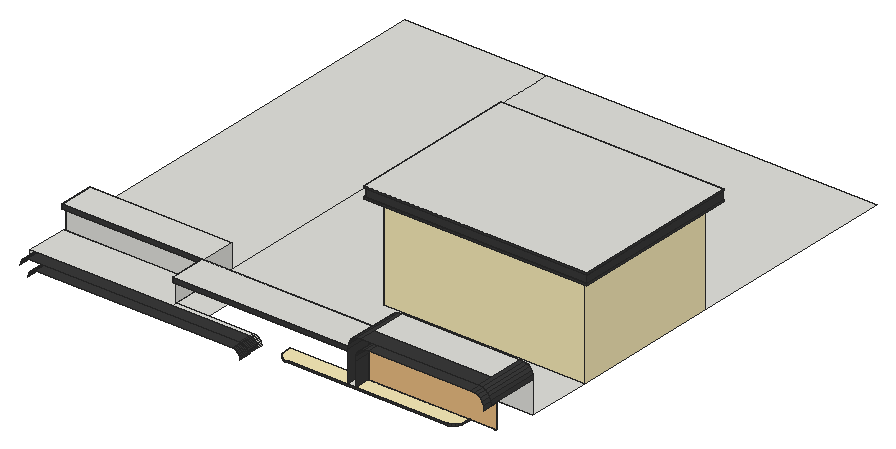
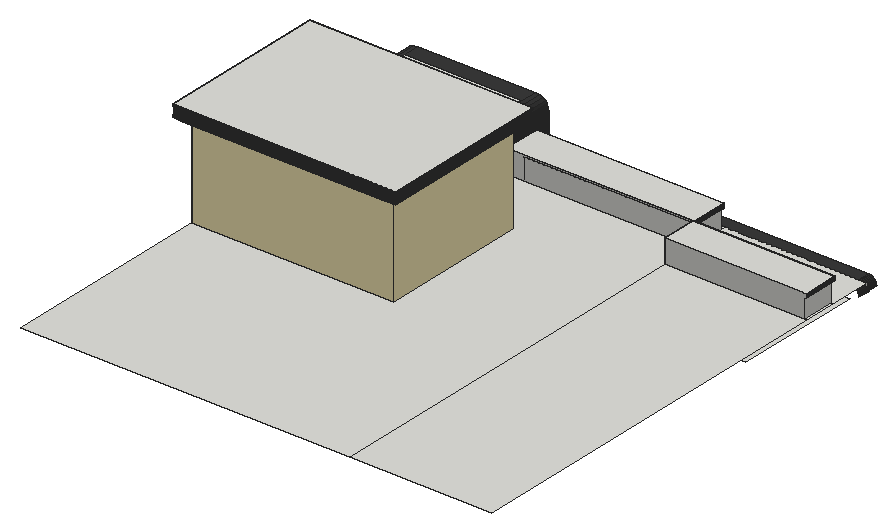
# SketchUp Ruby script. Lengths in inches.
U = 1.inch
M = Sketchup.active_model
def pt(a) = Geom::Point3d.new(a.map { |v| v * U })
def face(e, loops, mat)
  f = e.add_face(loops[0].map { |a| pt(a) })
  loops[1..].each { |l| e.add_face(l.map { |a| pt(a) }).erase! }
  f.material = f.back_material = mat if mat
  f
end
# faces: each face lists its corners as indices into pts; further lists are holes
def faces(e, pts, list, mat = nil) = list.each { |f| face(e, (f[0].is_a?(Array) ? f : [f]).map { |l| l.map { |i| pts[i] } }, mat) }
# xy, xz, yz: faces in a plane at the given z, y or x. An outline is a flat list of corners, or four numbers for a rectangle; further outlines are holes
def ring(l) = l.size == 4 ? [[l[0], l[1]], [l[2], l[1]], [l[2], l[3]], [l[0], l[3]]] : l.each_slice(2).to_a
def flat(e, list, mat, &to3) = list.each { |f| face(e, (f[0].is_a?(Array) ? f : [f]).map { |l| ring(l).map { |u, v| to3.(u, v) } }, mat) }
def xy(e, z, list, mat = nil) = flat(e, list, mat) { |x, y| [x, y, z] }
def xz(e, y, list, mat = nil) = flat(e, list, mat) { |x, z| [x, y, z] }
def yz(e, x, list, mat = nil) = flat(e, list, mat) { |y, z| [x, y, z] }
def lines(e, pts, list) = list.each { |a, b| e.add_line(pt(pts[a]), pt(pts[b])) }
# prism: a flat outline (further loops are holes) pulled along v
def prism(e, loops, v, mat = nil)
  f = face(e, loops, mat); d = Geom::Vector3d.new(v.map { |x| x * U })
  f.pushpull(f.normal.samedirection?(d) ? d.length : -d.length)
end
def box(e, o, s, mat = nil) = prism(e, [[o, [o[0] + s[0], o[1], o[2]], [o[0] + s[0], o[1] + s[1], o[2]], [o[0], o[1] + s[1], o[2]]]], [0, 0, s[2]], mat)
def at(x, y, z, deg = 0) = Geom::Transformation.translation(pt([x, y, z])) * Geom::Transformation.rotation(ORIGIN, Z_AXIS, deg.degrees)
def axes(o, x, y, z) = Geom::Transformation.new([*x, 0, *y, 0, *z, 0, *pt(o).to_a, 1])
def part(name) = M.definitions.add(name)
# library, detail: a bought-in or finely detailed component or shape, given as its bounding box
def library(name, o, s) = part(name).tap { |d| box(d.entities, o, s) }
def detail(e, o, s) = box(e.add_group.entities, o, s)
def put(e, d, t, mat = nil) = e.add_instance(d, t).tap { |i| i.material = mat if mat }
def group(e, t, mat = nil) = e.add_group.tap { |g| g.transformation = t; g.material = mat if mat }.entities
root = M.entities
M.materials.add("0899 AP 7833 SUNKISSED").color = [249, 236, 185]
M.materials.add("[Color M07]").color = [58, 58, 58]
M.materials.add("[Wood Veneer 02]").color = [190, 128, 91]
c1 = library("Group277\#1",[-65.14,-19,0],[130.28,38,0.24])
xy(root,243,[[9,135.1875,166.1,267.1875]])
xy(root,247,[[17,111.1875,217,123.1875]],"[Color M07]")
xy(root,253.0625,[[274.28,111.1875,432.47,111.1875,436.3,111.52,439.43,112.52,441.87,114.1875,443.61,116.52,444.65,119.52,445,123.1875,261.75,123.1875,262.1,119.52,263.14,116.52,264.88,114.1875,267.32,112.52,270.45,111.52]])
xy(root,255,[[334.71,111.1875,342.71,128.1875],[1,123.1875,145.5625,166.1875],[145.5625,123.1875,225,128.1875],[145.5625,164.1875,481,164.1875,481,230.0625,275.625,230.0625,275.625,382.59,481,382.59,481,601,145.5625,601],[1,166.1875,3,200.1875],
  [3,166.1875,145.5625,200.1875],[1,200.1875,145.5625,601],[275.625,230.0625,481,382.59]])
xy(root,255,[[274.28,111.1875,334.71,111.1875,334.71,128.1875,261.75,128.1875,261.75,123.1875,262.1,119.52,263.14,116.52,264.88,114.1875,267.32,112.52,270.45,111.52],[342.71,111.1875,432.47,111.1875,436.3,111.52,439.43,112.52,441.87,114.1875,443.61,116.52,444.65,119.52,445,123.1875,445,128.1875,342.71,128.1875]],"0899 AP 7833 SUNKISSED")
xy(root,255,[[9,111.1875,225,123.1875]],"[Color M07]")
xy(root,274.625,[[145.39,126.1875,144.83,126.24,144.37,126.39,144.02,126.64,143.77,127,143.61,127.45,143.5625,128.01,143.5625,164.1875,145.5625,164.1875,145.5625,128.1875,334.71,128.1875,334.71,126.1875],[1,164.1875,143.5625,166.1875],[143.5625,164.1875,145.5625,166.1875],[1,166.1875,3,200.1875]],"[Color M07]")
xy(root,277,[[145.5625,128.1875,317.59,164.1875]])
xy(root,279,[[145.39,126.1875,334.71,126.1875,334.71,164.1875,143.5625,164.1875,143.5625,128.01,143.61,127.45,143.77,127,144.02,126.64,144.37,126.39,144.83,126.24],[1,164.1875,145.5625,200.1875]])
xy(root,293,[[356.2,111.1875,459.51,128.1875]],"[Color M07]")
xy(root,301,[[348.2,128.1875,467.51,164.1875]])
xy(root,301,[[348.2,111.1875,467.51,128.1875]],"[Color M07]")
xy(root,352.4375,[[275.625,230.0625,481,382.59],[275.625,382.59,481,393.59]])
xy(root,352.4375,[[264.625,219.0625,264.625,393.59,275.625,393.59,275.625,230.0625,481,230.0625,481,393.59,492,393.59,492,219.0625]],"[Color M07]")
xy(root,354.4375,[[265.625,220.0625,491,392.59]])
xy(root,354.4375,[[264.625,219.0625,492,220.0625],[264.625,220.0625,265.625,393.59],[491,220.0625,492,393.59],[265.625,392.59,491,393.59]],"[Color M07]")
xy(root,362.4375,[[265.625,220.0625,491,392.59]])
xy(root,362.4375,[[264.625,219.0625,492,220.0625],[264.625,220.0625,265.625,393.59],[491,220.0625,492,393.59],[265.625,392.59,491,393.59]],"[Color M07]")
xy(root,364.4375,[[264.625,219.0625,492,393.59]])
xz(root,111.1875,[[274.28,253.0625,432.47,255]],"[Color M07]")
xz(root,123.1875,[[1,247,1.07,248.04,1.27,249.07,1.61,250.0625,2.07,251,2.65,251.87,3.34,252.66,4.13,253.35,5,253.93,5.9375,254.39,6.93,254.73,7.96,254.93,9,255,1,255]])
xz(root,126.1875,[[145.39,274.625,334.71,279]],"[Color M07]")
xz(root,128.1875,[[145.5625,274.625,317.59,277]])
xz(root,164.1875,[[145.5625,255,317.59,277],[317.59,255,317.59,279,334.71,279,334.71,287.51,335.09,291.63,336.21,295.01,338.08,297.63,340.71,299.5,344.08,300.625,348.2,301,467.51,301,471.63,300.625,475.01,299.5,477.63,297.63,479.5,295.01,480.625,291.63,481,287.51,481,255],[143.5625,274.625,145.5625,279],[145.5625,277,317.59,279]])
xz(root,164.1875,[[1,274.625,143.5625,279]],"[Color M07]")
xz(root,166.1875,[[3,255,145.5625,274.625]])
xz(root,200.1875,[[3,255,3,274.625,1,274.625,1,279,145.5625,279,145.5625,255]])
xz(root,219.0625,[[264.625,352.4375,492,354.4375],[264.625,362.4375,492,364.4375]],"[Color M07]")
xz(root,220.0625,[[265.625,354.4375,491,362.4375]],"[Color M07]")
xz(root,230.0625,[[275.625,255,481,352.4375]],"0899 AP 7833 SUNKISSED")
xz(root,382.59,[[275.625,255,481,352.4375]],"0899 AP 7833 SUNKISSED")
xz(root,392.59,[[265.625,354.4375,491,362.4375]],"[Color M07]")
xz(root,393.59,[[264.625,352.4375,492,354.4375],[264.625,362.4375,492,364.4375]],"[Color M07]")
yz(root,1,[[164.1875,274.625,200.1875,279]],"[Color M07]")
yz(root,3,[[166.1875,255,200.1875,274.625]])
yz(root,143.5625,[[128.01,274.625,164.1875,279]],"[Color M07]")
yz(root,145.5625,[[128.1875,255,164.1875,274.625],[164.1875,255,166.1875,274.625],[166.1875,255,200.1875,255,200.1875,279,164.1875,279,164.1875,274.625,166.1875,274.625],[128.1875,274.625,164.1875,277]])
yz(root,261.75,[[123.1875,253.0625,128.1875,255]],"[Color M07]")
yz(root,264.625,[[219.0625,352.4375,393.59,354.4375],[219.0625,362.4375,393.59,364.4375]],"[Color M07]")
yz(root,265.625,[[220.0625,354.4375,392.59,362.4375]],"[Color M07]")
yz(root,275.625,[[230.0625,255,382.59,352.4375]],"0899 AP 7833 SUNKISSED")
yz(root,334.71,[[126.1875,274.625,128.1875,279]])
yz(root,334.71,[[111.1875,255,111.1875,287.51,164.1875,287.51,164.1875,279,126.1875,279,126.1875,274.625,128.1875,274.625,128.1875,255]],"[Color M07]")
yz(root,342.71,[[111.1875,255,128.1875,279.51]],"[Color M07]")
yz(root,445,[[123.1875,253.0625,128.1875,255]],"[Color M07]")
yz(root,481,[[230.0625,255,382.59,352.4375]],"0899 AP 7833 SUNKISSED")
yz(root,491,[[220.0625,354.4375,392.59,362.4375]],"[Color M07]")
yz(root,492,[[219.0625,352.4375,393.59,354.4375],[219.0625,362.4375,393.59,364.4375]],"[Color M07]")
p = [[9,123.1875,239],[9.07,123.1875,240.04],[9.07,111.1875,240.04],[9,111.1875,239],[224.93,123.1875,240.04],[225,123.1875,239],
  [225,111.1875,239],[224.93,111.1875,240.04],[9.27,123.1875,241.07],[9.27,111.1875,241.07],[224.73,123.1875,241.07],[224.73,111.1875,241.07],
  [9.61,123.1875,242.0625],[9.61,111.1875,242.0625],[224.39,123.1875,242.0625],[224.39,111.1875,242.0625],[10.07,123.1875,243],[10.07,111.1875,243],
  [223.93,123.1875,243],[223.93,111.1875,243],[10.65,123.1875,243.87],[10.65,111.1875,243.87],[223.35,123.1875,243.87],[223.35,111.1875,243.87],
  [11.34,123.1875,244.66],[11.34,111.1875,244.66],[222.66,123.1875,244.66],[222.66,111.1875,244.66],[12.13,123.1875,245.35],[12.13,111.1875,245.35],
  [221.87,123.1875,245.35],[221.87,111.1875,245.35],[13,123.1875,245.93],[13,111.1875,245.93],[221,123.1875,245.93],[221,111.1875,245.93],
  [13.9375,123.1875,246.39],[13.9375,111.1875,246.39],[220.0625,123.1875,246.39],[220.0625,111.1875,246.39],[14.93,123.1875,246.73],[14.93,111.1875,246.73],
  [219.07,123.1875,246.73],[219.07,111.1875,246.73],[15.96,123.1875,246.93],[15.96,111.1875,246.93],[218.04,123.1875,246.93],[218.04,111.1875,246.93],
  [17,123.1875,247],[17,111.1875,247],[217,123.1875,247],[217,111.1875,247],[1.07,123.1875,248.04],[1,123.1875,247],
  [1,111.1875,247],[1.07,111.1875,248.04],[233,123.1875,247],[232.93,123.1875,248.04],[232.93,111.1875,248.04],[233,111.1875,247],
  [233,128.1875,247],[232.93,128.1875,248.04],[1.27,123.1875,249.07],[1.27,111.1875,249.07],[232.73,123.1875,249.07],[232.73,111.1875,249.07],
  [232.73,128.1875,249.07],[1.61,123.1875,250.0625],[1.61,111.1875,250.0625],[232.39,123.1875,250.0625],[232.39,111.1875,250.0625],[232.39,128.1875,250.0625],
  [2.07,123.1875,251],[2.07,111.1875,251],[231.93,123.1875,251],[231.93,111.1875,251],[231.93,128.1875,251],[2.65,123.1875,251.87],
  [2.65,111.1875,251.87],[231.35,123.1875,251.87],[231.35,111.1875,251.87],[231.35,128.1875,251.87],[3.34,123.1875,252.66],[3.34,111.1875,252.66],
  [230.66,123.1875,252.66],[230.66,111.1875,252.66],[230.66,128.1875,252.66],[4.13,123.1875,253.35],[4.13,111.1875,253.35],[229.87,123.1875,253.35],
  [229.87,111.1875,253.35],[229.87,128.1875,253.35],[270.45,111.52,255],[270.45,111.52,253.0625],[274.28,111.1875,253.0625],[274.28,111.1875,255],
  [432.47,111.1875,255],[432.47,111.1875,253.0625],[436.3,111.52,253.0625],[436.3,111.52,255],[267.32,112.52,255],[267.32,112.52,253.0625],
  [439.43,112.52,253.0625],[439.43,112.52,255],[264.88,114.1875,255],[264.88,114.1875,253.0625],[441.87,114.1875,253.0625],[441.87,114.1875,255],
  [263.14,116.52,255],[263.14,116.52,253.0625],[443.61,116.52,253.0625],[443.61,116.52,255],[262.1,119.52,255],[262.1,119.52,253.0625],
  [444.65,119.52,253.0625],[444.65,119.52,255],[261.75,123.1875,255],[261.75,123.1875,253.0625],[445,123.1875,253.0625],[445,123.1875,255],
  [5,123.1875,253.93],[5,111.1875,253.93],[229,123.1875,253.93],[229,111.1875,253.93],[229,128.1875,253.93],[5.9375,123.1875,254.39],
  [5.9375,111.1875,254.39],[228.0625,123.1875,254.39],[228.0625,111.1875,254.39],[228.0625,128.1875,254.39],[6.93,123.1875,254.73],[6.93,111.1875,254.73],
  [227.07,123.1875,254.73],[227.07,111.1875,254.73],[227.07,128.1875,254.73],[7.96,123.1875,254.93],[7.96,111.1875,254.93],[226.04,123.1875,254.93],
  [226.04,111.1875,254.93],[226.04,128.1875,254.93],[9,123.1875,255],[9,111.1875,255],[225,123.1875,255],[225,111.1875,255],
  [225,128.1875,255],[144.37,126.39,279],[144.37,126.39,274.625],[144.83,126.24,274.625],[144.83,126.24,279],[145.39,126.1875,274.625],
  [145.39,126.1875,279],[144.02,126.64,279],[144.02,126.64,274.625],[143.77,127,279],[143.77,127,274.625],[143.61,127.45,279],
  [143.61,127.45,274.625],[143.5625,128.01,279],[143.5625,128.01,274.625],[342.71,111.1875,279.51],[342.71,128.1875,279.51],[343.09,128.1875,283.63],
  [343.09,111.1875,283.63],[472.625,111.1875,283.63],[472.625,128.1875,283.63],[473,128.1875,279.51],[473,111.1875,279.51],[344.21,128.1875,287.01],
  [344.21,111.1875,287.01],[471.5,111.1875,287.01],[471.5,128.1875,287.01],[346.08,128.1875,289.63],[346.08,111.1875,289.63],[469.63,111.1875,289.63],
  [469.63,128.1875,289.63],[334.71,164.1875,287.51],[334.71,111.1875,287.51],[335.09,111.1875,291.63],[335.09,164.1875,291.63],[480.625,164.1875,291.63],
  [480.625,111.1875,291.63],[481,111.1875,287.51],[481,128.1875,287.51],[481,164.1875,287.51],[348.71,128.1875,291.5],[348.71,111.1875,291.5],
  [467.01,111.1875,291.5],[467.01,128.1875,291.5],[352.08,128.1875,292.625],[352.08,111.1875,292.625],[463.63,111.1875,292.625],[463.63,128.1875,292.625],
  [336.21,111.1875,295.01],[336.21,164.1875,295.01],[479.5,164.1875,295.01],[479.5,111.1875,295.01],[356.2,128.1875,293],[356.2,111.1875,293],
  [459.51,111.1875,293],[459.51,128.1875,293],[338.08,111.1875,297.63],[338.08,164.1875,297.63],[477.63,164.1875,297.63],[477.63,111.1875,297.63],
  [340.71,111.1875,299.5],[340.71,164.1875,299.5],[475.01,164.1875,299.5],[475.01,111.1875,299.5],[344.08,111.1875,300.625],[344.08,164.1875,300.625],
  [471.63,164.1875,300.625],[471.63,111.1875,300.625],[348.2,111.1875,301],[348.2,128.1875,301],[348.2,164.1875,301],[467.51,128.1875,301],
  [467.51,111.1875,301],[467.51,164.1875,301],[317.59,128.1875,277],[317.59,128.1875,279],[445,128.1875,255],[473,128.1875,255]]
faces(root,p,[[0,1,2,3],[4,5,6,7],[1,8,9,2],[10,4,7,11],[8,12,13,9],[14,10,11,15],[12,16,17,13],[18,14,15,19],
  [16,20,21,17],[22,18,19,23],[20,24,25,21],[26,22,23,27],[24,28,29,25],[30,26,27,31],[28,32,33,29],[34,30,31,35],
  [32,36,37,33],[38,34,35,39],[36,40,41,37],[42,38,39,43],[40,44,45,41],[46,42,43,47],[44,48,49,45],[50,46,47,51],
  [52,53,54,55],[56,57,58,59],[62,52,55,63],[57,64,65,58],[67,62,63,68],[64,69,70,65],[72,67,68,73],[69,74,75,70],
  [77,72,73,78],[74,79,80,75],[82,77,78,83],[79,84,85,80],[87,82,83,88],[84,89,90,85],[92,93,94,95],[96,97,98,99],
  [100,101,93,92],[99,98,102,103],[104,105,101,100],[106,107,103,102],[108,109,105,104],[107,106,110,111],[112,113,109,108],[111,110,114,115],
  [116,117,113,112],[118,119,115,114],[120,87,88,121],[89,122,123,90],[125,120,121,126],[122,127,128,123],[130,125,126,131],[127,132,133,128],
  [135,130,131,136],[132,137,138,133],[140,135,136,141],[137,142,143,138],[145,146,147,148],[148,147,149,150],[151,152,146,145],[153,154,152,151],
  [155,156,154,153],[157,158,156,155],[159,160,161,162],[163,164,165,166],[162,161,167,168],[169,170,164,163],[168,167,171,172],[173,174,170,169],
  [175,176,177,178],[179,180,181,182,183],[172,171,184,185],[186,187,174,173],[185,184,188,189],[190,191,187,186],[178,177,192,193],[194,195,180,179],
  [189,188,196,197],[198,199,191,190],[193,192,200,201],[202,203,195,194],[201,200,204,205],[206,207,203,202],[205,204,208,209],[210,211,207,206],
  [209,208,212,213,214],[215,216,211,210,217]],"[Color M07]")
faces(root,p,[[57,56,60,61],[64,57,61,66],[69,64,66,71],[74,69,71,76],[79,74,76,81],[84,79,81,86],[89,84,86,91],[122,89,91,124],
  [127,122,124,129],[132,127,129,134],[137,132,134,139],[142,137,139,144]])
lines(root,p,[[218,219],[220,221]])
put(root,c1,axes([407.86,128.1875,274],[1,0,0],[0,0,1],[0,-1,0]),"[Wood Veneer 02]")
